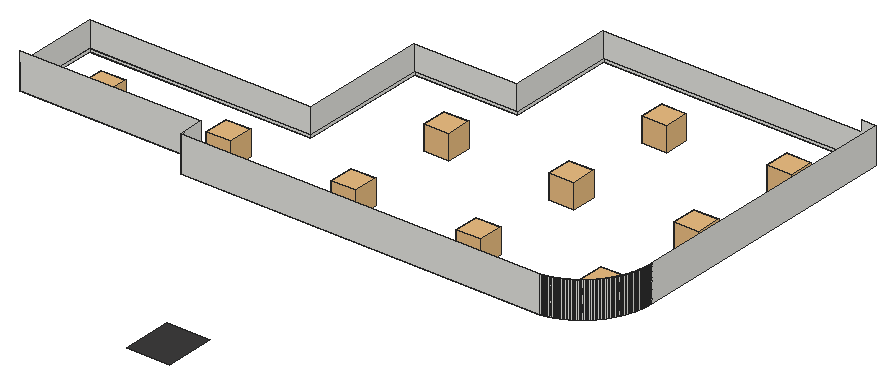
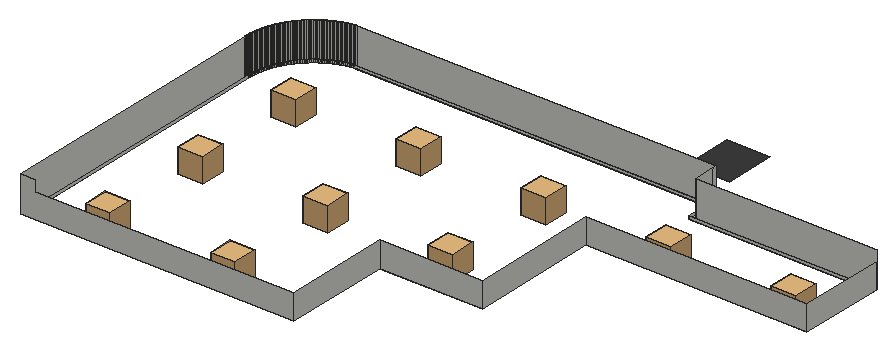
# SketchUp Ruby script. Lengths in inches.
U = 1.inch
M = Sketchup.active_model
def pt(a) = Geom::Point3d.new(a.map { |v| v * U })
def face(e, loops, mat)
  f = e.add_face(loops[0].map { |a| pt(a) })
  loops[1..].each { |l| e.add_face(l.map { |a| pt(a) }).erase! }
  f.material = f.back_material = mat if mat
  f
end
# faces: each face lists its corners as indices into pts; further lists are holes
def faces(e, pts, list, mat = nil) = list.each { |f| face(e, (f[0].is_a?(Array) ? f : [f]).map { |l| l.map { |i| pts[i] } }, mat) }
# xy, xz, yz: faces in a plane at the given z, y or x. An outline is a flat list of corners, or four numbers for a rectangle; further outlines are holes
def ring(l) = l.size == 4 ? [[l[0], l[1]], [l[2], l[1]], [l[2], l[3]], [l[0], l[3]]] : l.each_slice(2).to_a
def flat(e, list, mat, &to3) = list.each { |f| face(e, (f[0].is_a?(Array) ? f : [f]).map { |l| ring(l).map { |u, v| to3.(u, v) } }, mat) }
def xy(e, z, list, mat = nil) = flat(e, list, mat) { |x, y| [x, y, z] }
def xz(e, y, list, mat = nil) = flat(e, list, mat) { |x, z| [x, y, z] }
def yz(e, x, list, mat = nil) = flat(e, list, mat) { |y, z| [x, y, z] }
def lines(e, pts, list) = list.each { |a, b| e.add_line(pt(pts[a]), pt(pts[b])) }
# prism: a flat outline (further loops are holes) pulled along v
def prism(e, loops, v, mat = nil)
  f = face(e, loops, mat); d = Geom::Vector3d.new(v.map { |x| x * U })
  f.pushpull(f.normal.samedirection?(d) ? d.length : -d.length)
end
def box(e, o, s, mat = nil) = prism(e, [[o, [o[0] + s[0], o[1], o[2]], [o[0] + s[0], o[1] + s[1], o[2]], [o[0], o[1] + s[1], o[2]]]], [0, 0, s[2]], mat)
def at(x, y, z, deg = 0) = Geom::Transformation.translation(pt([x, y, z])) * Geom::Transformation.rotation(ORIGIN, Z_AXIS, deg.degrees)
def axes(o, x, y, z) = Geom::Transformation.new([*x, 0, *y, 0, *z, 0, *pt(o).to_a, 1])
def part(name) = M.definitions.add(name)
# library, detail: a bought-in or finely detailed component or shape, given as its bounding box
def library(name, o, s) = part(name).tap { |d| box(d.entities, o, s) }
def detail(e, o, s) = box(e.add_group.entities, o, s)
def put(e, d, t, mat = nil) = e.add_instance(d, t).tap { |i| i.material = mat if mat }
def group(e, t, mat = nil) = e.add_group.tap { |g| g.transformation = t; g.material = mat if mat }.entities
root = M.entities
M.materials.add("[Granite Dark Gray]").color = [61, 60, 60]
c1 = library("3",[-4.91,-4.91,-13.58],[13.82,13.82,13.58])
xy(root,75,[[168,58,192,86]],"[Granite Dark Gray]")
xy(root,106,[[[124.5,150,124.5,164,24,164,24,212,147,212,147,284,204,284,204,344,356,344,356,187.02,355.99,186.68,355.99,186.34,355.97,186.01,355.96,185.67,355.94,185.34,355.9,184.66,355.87,184.33,355.84,183.99,355.81,183.66,355.77,183.32,355.74,182.99,355.69,182.65,355.65,182.32,355.55,181.66,355.5,181.32,355.26,180,355.1875,179.67,355.12,179.34,355.04,179.01,354.97,178.68,354.89,178.36,354.81,178.03,354.72,177.7,354.54,177.06,354.45,176.73,354.15,175.77,353.93,175.13,353.82,174.8125,353.71,174.49,353.59,174.18,353.47,173.86,353.23,173.24,352.84,172.31,352.56,171.69,352.42,171.39,352.28,171.08,351.83,170.18,351.35,169.28,351.03,168.7,350.86,168.4,350.6875,168.11,350.52,167.83,350.16,167.25,349.98,166.97,349.8,166.6875,349.61,166.4,349.23,165.85,349.04,165.57,348.85,165.3,348.45,164.76,348.24,164.49,348.04,164.22,347.83,163.95,347.2,163.17,346.98,162.91,346.76,162.66,346.54,162.4,346.32,162.15,345.86,161.65,345.63,161.41,345.4,161.16,345.17,160.92,344.93,160.68,344.69,160.45,344.45,160.21,344.21,159.98,343.96,159.75,343.72,159.52,343.47,159.29,343.22,159.07,342.96,158.84,342.71,158.625,342.45,158.41,342.19,158.19,341.41,157.56,341.14,157.35,340.06,156.55,339.5,156.17,339.23,155.98,338.95,155.79,338.66,155.6,338.1,155.24,337.81,155.07,337.52,154.89,336.94,154.55,336.65,154.39,336.35,154.22,336.06,154.0625,335.76,153.9,335.46,153.75,335.16,153.59,334.86,153.44,334.5625,153.29,334.26,153.15,333.95,153.01,333.65,152.87,333.03,152.59,332.41,152.33,332.1,152.21,331.78,152.08,331.47,151.96,331.15,151.85,330.84,151.73,329.88,151.4,329.5625,151.3,329.24,151.2,328.6,151,328.27,150.91,327.95,150.82,327.625,150.73,327.3,150.65,326.64,150.49,326.31,150.42,325.99,150.34,325.66,150.28,325.33,150.21,325,150.15,324.66,150.09,324.17,150],[126.5,152,324,152,324.3125,152.05,324.63,152.11,325.25,152.23,325.57,152.3,325.88,152.37,326.1875,152.44,326.5,152.51,327.43,152.75,327.73,152.84,328.04,152.92,328.35,153.01,328.65,153.11,328.95,153.2,329.26,153.3,329.56,153.4,329.86,153.51,330.16,153.61,330.76,153.83,331.06,153.95,331.36,154.06,331.65,154.18,331.95,154.31,332.24,154.43,332.53,154.56,332.82,154.6875,333.11,154.82,333.4,154.96,333.6875,155.09,333.98,155.23,334.26,155.38,334.54,155.52,334.83,155.67,335.39,155.97,335.67,156.13,335.94,156.29,336.22,156.45,336.49,156.61,336.77,156.77,337.58,157.28,337.84,157.46,338.11,157.63,338.375,157.8125,338.64,158,338.9,158.18,339.15,158.37,339.41,158.55,339.67,158.75,339.92,158.9375,340.17,159.13,340.92,159.73,341.16,159.9375,341.41,160.14,341.65,160.35,341.89,160.5625,342.125,160.77,342.36,160.99,342.6,161.21,343.29,161.87,343.74,162.32,344.4,163.01,344.61,163.25,344.83,163.49,345.04,163.72,345.25,163.96,345.45,164.21,345.66,164.45,345.86,164.7,346.0625,164.94,346.26,165.19,346.46,165.44,346.65,165.7,346.84,165.95,347.41,166.73,347.77,167.25,347.95,167.52,348.125,167.78,348.3,168.05,348.64,168.59,348.8,168.86,348.97,169.13,349.13,169.41,349.29,169.6875,349.45,169.96,349.75,170.52,349.9,170.81,350.05,171.09,350.19,171.37,350.47,171.95,350.61,172.23,350.74,172.52,350.875,172.8125,351,173.11,351.13,173.4,351.25,173.69,351.37,173.99,351.49,174.28,351.61,174.58,351.83,175.18,351.9375,175.48,352.04,175.78,352.15,176.08,352.25,176.38,352.34,176.6875,352.4375,176.99,352.53,177.3,352.62,177.6,352.7,177.91,352.79,178.22,352.95,178.84,353.3,180.39,353.36,180.71,353.42,181.02,353.47,181.33,353.53,181.65,353.58,181.96,353.625,182.28,353.67,182.59,353.75,183.23,353.79,183.54,353.88,184.5,353.9,184.8125,353.93,185.13,353.95,185.45,353.96,185.77,353.98,186.09,353.99,186.41,354,186.72,354,342,206,342,206,282,149,282,149,210,26,210,26,166,126.5,166]]])
xz(root,150,[[124.5,106,324.17,126]])
xz(root,152,[[126.5,106,324,107.5]])
xz(root,164,[[24,106,124.5,126]])
xz(root,166,[[26,106,126.5,107.5]])
xz(root,210,[[26,106,149,107.5]])
xz(root,212,[[24,106,147,120]])
xz(root,282,[[149,106,206,107.5]])
xz(root,284,[[147,106,204,120]])
xz(root,342,[[206,106,354,107.5]])
xz(root,344,[[204,106,204,120,348,120,348,126,356,126,356,106]])
yz(root,24,[[164,106,212,120]])
yz(root,26,[[166,106,210,107.5]])
yz(root,124.5,[[150,106,152,126],[152,106,164,126]])
yz(root,126.5,[[152,106,166,107.5]])
yz(root,147,[[212,106,284,120]])
yz(root,149,[[210,106,282,107.5]])
yz(root,204,[[284,106,344,120]])
yz(root,206,[[282,106,342,107.5]])
yz(root,354,[[186.72,106,187.04,107.5],[187.04,106,187.36,107.5],[187.36,106,187.68,107.5],[187.68,106,188,107.5],[188,106,342,107.5]])
yz(root,355.99,[[186.34,106,186.68,126]])
yz(root,356,[[187.02,106,187.35,126],[187.35,106,187.69,126],[187.69,106,188.01,126],[188.01,106,344,126]])
p = [[324.66,150.09,126],[324.17,150,126],[324.17,150,106],[324.66,150.09,106],[325,150.15,126],[325,150.15,106],
  [325.33,150.21,126],[325.33,150.21,106],[325.66,150.28,126],[325.66,150.28,106],[325.99,150.34,126],[325.99,150.34,106],
  [326.31,150.42,126],[326.31,150.42,106],[326.64,150.49,126],[326.64,150.49,106],[326.97,150.57,126],[326.97,150.57,106],
  [327.3,150.65,126],[327.3,150.65,106],[327.625,150.73,126],[327.625,150.73,106],[327.95,150.82,126],[327.95,150.82,106],
  [328.27,150.91,126],[328.27,150.91,106],[328.6,151,126],[328.6,151,106],[328.92,151.1,126],[328.92,151.1,106],
  [329.24,151.2,126],[329.24,151.2,106],[329.5625,151.3,126],[329.5625,151.3,106],[329.88,151.4,126],[329.88,151.4,106],
  [330.2,151.51,126],[330.2,151.51,106],[330.52,151.62,126],[330.52,151.62,106],[330.84,151.73,126],[330.84,151.73,106],
  [331.15,151.85,126],[331.15,151.85,106],[331.47,151.96,126],[331.47,151.96,106],[324,152,107.5],[324.3125,152.05,107.5],
  [324.3125,152.05,106],[324,152,106],[331.78,152.08,126],[331.78,152.08,106],[324.63,152.11,107.5],[324.63,152.11,106],
  [324.94,152.17,107.5],[324.94,152.17,106],[332.1,152.21,126],[332.1,152.21,106],[325.25,152.23,107.5],[325.25,152.23,106],
  [325.57,152.3,107.5],[325.57,152.3,106],[332.41,152.33,126],[332.41,152.33,106],[325.88,152.37,107.5],[325.88,152.37,106],
  [332.72,152.46,126],[332.72,152.46,106],[326.1875,152.44,107.5],[326.1875,152.44,106],[326.5,152.51,107.5],[326.5,152.51,106],
  [326.81,152.59,107.5],[326.81,152.59,106],[333.03,152.59,126],[333.03,152.59,106],[327.12,152.67,107.5],[327.12,152.67,106],
  [333.34,152.73,126],[333.34,152.73,106],[327.43,152.75,107.5],[327.43,152.75,106],[333.65,152.87,126],[333.65,152.87,106],
  [327.73,152.84,107.5],[327.73,152.84,106],[328.04,152.92,107.5],[328.04,152.92,106],[328.35,153.01,107.5],[328.35,153.01,106],
  [333.95,153.01,126],[333.95,153.01,106],[328.65,153.11,107.5],[328.65,153.11,106],[334.26,153.15,126],[334.26,153.15,106],
  [328.95,153.2,107.5],[328.95,153.2,106],[334.5625,153.29,126],[334.5625,153.29,106],[329.26,153.3,107.5],[329.26,153.3,106],
  [329.56,153.4,107.5],[329.56,153.4,106],[334.86,153.44,126],[334.86,153.44,106],[329.86,153.51,107.5],[329.86,153.51,106],
  [335.16,153.59,126],[335.16,153.59,106],[330.16,153.61,107.5],[330.16,153.61,106],[330.46,153.72,107.5],[330.46,153.72,106],
  [335.46,153.75,126],[335.46,153.75,106],[330.76,153.83,107.5],[330.76,153.83,106],[335.76,153.9,126],[335.76,153.9,106],
  [331.06,153.95,107.5],[331.06,153.95,106],[331.36,154.06,107.5],[331.36,154.06,106],[336.06,154.0625,126],[336.06,154.0625,106],
  [331.65,154.18,107.5],[331.65,154.18,106],[336.35,154.22,126],[336.35,154.22,106],[331.95,154.31,107.5],[331.95,154.31,106],
  [336.65,154.39,126],[336.65,154.39,106],[332.24,154.43,107.5],[332.24,154.43,106],[332.53,154.56,107.5],[332.53,154.56,106],
  [336.94,154.55,126],[336.94,154.55,106],[332.82,154.6875,107.5],[332.82,154.6875,106],[337.23,154.72,126],[337.23,154.72,106],
  [333.11,154.82,107.5],[333.11,154.82,106],[337.52,154.89,126],[337.52,154.89,106],[333.4,154.96,107.5],[333.4,154.96,106],
  [337.81,155.07,126],[337.81,155.07,106],[333.6875,155.09,107.5],[333.6875,155.09,106],[333.98,155.23,107.5],[333.98,155.23,106],
  [338.1,155.24,126],[338.1,155.24,106],[334.26,155.38,107.5],[334.26,155.38,106],[338.38,155.42,126],[338.38,155.42,106],
  [334.54,155.52,107.5],[334.54,155.52,106],[338.66,155.6,126],[338.66,155.6,106],[334.83,155.67,107.5],[334.83,155.67,106],
  [338.95,155.79,126],[338.95,155.79,106],[335.11,155.82,107.5],[335.11,155.82,106],[335.39,155.97,107.5],[335.39,155.97,106],
  [339.23,155.98,126],[339.23,155.98,106],[335.67,156.13,107.5],[335.67,156.13,106],[339.5,156.17,126],[339.5,156.17,106],
  [335.94,156.29,107.5],[335.94,156.29,106],[339.78,156.36,126],[339.78,156.36,106],[336.22,156.45,107.5],[336.22,156.45,106],
  [336.49,156.61,107.5],[336.49,156.61,106],[340.06,156.55,126],[340.06,156.55,106],[336.77,156.77,107.5],[336.77,156.77,106],
  [340.33,156.75,126],[340.33,156.75,106],[340.6,156.95,126],[340.6,156.95,106],[337.04,156.94,107.5],[337.04,156.94,106],
  [337.31,157.11,107.5],[337.31,157.11,106],[340.87,157.15,126],[340.87,157.15,106],[337.58,157.28,107.5],[337.58,157.28,106],
  [341.14,157.35,126],[341.14,157.35,106],[337.84,157.46,107.5],[337.84,157.46,106],[341.41,157.56,126],[341.41,157.56,106],
  [338.11,157.63,107.5],[338.11,157.63,106],[338.375,157.8125,107.5],[338.375,157.8125,106],[341.67,157.77,126],[341.67,157.77,106],
  [338.64,158,107.5],[338.64,158,106],[341.93,157.98,126],[341.93,157.98,106],[338.9,158.18,107.5],[338.9,158.18,106],
  [342.19,158.19,126],[342.19,158.19,106],[339.15,158.37,107.5],[339.15,158.37,106],[342.45,158.41,126],[342.45,158.41,106],
  [339.41,158.55,107.5],[339.41,158.55,106],[342.71,158.625,126],[342.71,158.625,106],[339.67,158.75,107.5],[339.67,158.75,106],
  [342.96,158.84,126],[342.96,158.84,106],[339.92,158.9375,107.5],[339.92,158.9375,106],[343.22,159.07,126],[343.22,159.07,106],
  [340.17,159.13,107.5],[340.17,159.13,106],[340.42,159.33,107.5],[340.42,159.33,106],[343.47,159.29,126],[343.47,159.29,106],
  [340.67,159.53,107.5],[340.67,159.53,106],[343.72,159.52,126],[343.72,159.52,106],[340.92,159.73,107.5],[340.92,159.73,106],
  [343.96,159.75,126],[343.96,159.75,106],[341.16,159.9375,107.5],[341.16,159.9375,106],[344.21,159.98,126],[344.21,159.98,106],
  [341.41,160.14,107.5],[341.41,160.14,106],[344.45,160.21,126],[344.45,160.21,106],[341.65,160.35,107.5],[341.65,160.35,106],
  [344.69,160.45,126],[344.69,160.45,106],[341.89,160.5625,107.5],[341.89,160.5625,106],[344.93,160.68,126],[344.93,160.68,106],
  [342.125,160.77,107.5],[342.125,160.77,106],[345.17,160.92,126],[345.17,160.92,106],[342.36,160.99,107.5],[342.36,160.99,106],
  [345.4,161.16,126],[345.4,161.16,106],[342.6,161.21,107.5],[342.6,161.21,106],[342.83,161.43,107.5],[342.83,161.43,106],
  [345.63,161.41,126],[345.63,161.41,106],[343.06,161.65,107.5],[343.06,161.65,106],[345.86,161.65,126],[345.86,161.65,106],
  [343.29,161.87,107.5],[343.29,161.87,106],[346.09,161.9,126],[346.09,161.9,106],[343.51,162.09,107.5],[343.51,162.09,106],
  [346.32,162.15,126],[346.32,162.15,106],[343.74,162.32,107.5],[343.74,162.32,106],[346.54,162.4,126],[346.54,162.4,106],
  [343.96,162.55,107.5],[343.96,162.55,106],[346.76,162.66,126],[346.76,162.66,106],[344.18,162.78,107.5],[344.18,162.78,106],
  [346.98,162.91,126],[346.98,162.91,106],[344.4,163.01,107.5],[344.4,163.01,106],[347.2,163.17,126],[347.2,163.17,106],
  [344.61,163.25,107.5],[344.61,163.25,106],[344.83,163.49,107.5],[344.83,163.49,106],[347.41,163.43,126],[347.41,163.43,106],
  [347.62,163.69,126],[347.62,163.69,106],[345.04,163.72,107.5],[345.04,163.72,106],[345.25,163.96,107.5],[345.25,163.96,106],
  [347.83,163.95,126],[347.83,163.95,106],[345.45,164.21,107.5],[345.45,164.21,106],[348.04,164.22,126],[348.04,164.22,106],
  [345.66,164.45,107.5],[345.66,164.45,106],[348.24,164.49,126],[348.24,164.49,106],[345.86,164.7,107.5],[345.86,164.7,106],
  [348.45,164.76,126],[348.45,164.76,106],[346.0625,164.94,107.5],[346.0625,164.94,106],[348.65,165.03,126],[348.65,165.03,106],
  [346.26,165.19,107.5],[346.26,165.19,106],[348.85,165.3,126],[348.85,165.3,106],[346.46,165.44,107.5],[346.46,165.44,106],
  [349.04,165.57,126],[349.04,165.57,106],[346.65,165.7,107.5],[346.65,165.7,106],[349.23,165.85,126],[349.23,165.85,106],
  [346.84,165.95,107.5],[346.84,165.95,106],[349.42,166.125,126],[349.42,166.125,106],[347.03,166.21,107.5],[347.03,166.21,106],
  [349.61,166.4,126],[349.61,166.4,106],[347.22,166.47,107.5],[347.22,166.47,106],[349.8,166.6875,126],[349.8,166.6875,106],
  [347.41,166.73,107.5],[347.41,166.73,106],[347.59,166.99,107.5],[347.59,166.99,106],[349.98,166.97,126],[349.98,166.97,106],
  [347.77,167.25,107.5],[347.77,167.25,106],[350.16,167.25,126],[350.16,167.25,106],[347.95,167.52,107.5],[347.95,167.52,106],
  [350.34,167.54,126],[350.34,167.54,106],[348.125,167.78,107.5],[348.125,167.78,106],[350.52,167.83,126],[350.52,167.83,106],
  [348.3,168.05,107.5],[348.3,168.05,106],[350.6875,168.11,126],[350.6875,168.11,106],[348.47,168.32,107.5],[348.47,168.32,106],
  [350.86,168.4,126],[350.86,168.4,106],[348.64,168.59,107.5],[348.64,168.59,106],[351.03,168.7,126],[351.03,168.7,106],
  [348.8,168.86,107.5],[348.8,168.86,106],[351.19,168.99,126],[351.19,168.99,106],[348.97,169.13,107.5],[348.97,169.13,106],
  [351.35,169.28,126],[351.35,169.28,106],[349.13,169.41,107.5],[349.13,169.41,106],[351.51,169.58,126],[351.51,169.58,106],
  [349.29,169.6875,107.5],[349.29,169.6875,106],[351.67,169.88,126],[351.67,169.88,106],[349.45,169.96,107.5],[349.45,169.96,106],
  [351.83,170.18,126],[351.83,170.18,106],[349.6,170.24,107.5],[349.6,170.24,106],[349.75,170.52,107.5],[349.75,170.52,106],
  [351.98,170.48,126],[351.98,170.48,106],[349.9,170.81,107.5],[349.9,170.81,106],[352.13,170.78,126],[352.13,170.78,106],
  [350.05,171.09,107.5],[350.05,171.09,106],[352.28,171.08,126],[352.28,171.08,106],[350.19,171.37,107.5],[350.19,171.37,106],
  [352.42,171.39,126],[352.42,171.39,106],[350.33,171.66,107.5],[350.33,171.66,106],[352.56,171.69,126],[352.56,171.69,106],
  [350.47,171.95,107.5],[350.47,171.95,106],[352.7,172,126],[352.7,172,106],[350.61,172.23,107.5],[350.61,172.23,106],
  [352.84,172.31,126],[352.84,172.31,106],[350.74,172.52,107.5],[350.74,172.52,106],[352.97,172.62,126],[352.97,172.62,106],
  [350.875,172.8125,107.5],[350.875,172.8125,106],[353.1,172.93,126],[353.1,172.93,106],[351,173.11,107.5],[351,173.11,106],
  [353.23,173.24,126],[353.23,173.24,106],[351.13,173.4,107.5],[351.13,173.4,106],[353.35,173.55,126],[353.35,173.55,106],
  [351.25,173.69,107.5],[351.25,173.69,106],[353.47,173.86,126],[353.47,173.86,106],[351.37,173.99,107.5],[351.37,173.99,106],
  [353.59,174.18,126],[353.59,174.18,106],[351.49,174.28,107.5],[351.49,174.28,106],[353.71,174.49,126],[353.71,174.49,106],
  [351.61,174.58,107.5],[351.61,174.58,106],[353.82,174.8125,126],[353.82,174.8125,106],[351.72,174.88,107.5],[351.72,174.88,106],
  [353.93,175.13,126],[353.93,175.13,106],[351.83,175.18,107.5],[351.83,175.18,106],[354.04,175.45,126],[354.04,175.45,106],
  [351.9375,175.48,107.5],[351.9375,175.48,106],[354.15,175.77,126],[354.15,175.77,106],[352.04,175.78,107.5],[352.04,175.78,106],
  [352.15,176.08,107.5],[352.15,176.08,106],[354.25,176.09,126],[354.25,176.09,106],[352.25,176.38,107.5],[352.25,176.38,106],
  [354.35,176.41,126],[354.35,176.41,106],[352.34,176.6875,107.5],[352.34,176.6875,106],[354.45,176.73,126],[354.45,176.73,106],
  [352.4375,176.99,107.5],[352.4375,176.99,106],[354.54,177.06,126],[354.54,177.06,106],[352.53,177.3,107.5],[352.53,177.3,106],
  [354.63,177.38,126],[354.63,177.38,106],[352.62,177.6,107.5],[352.62,177.6,106],[354.72,177.7,126],[354.72,177.7,106],
  [352.7,177.91,107.5],[352.7,177.91,106],[354.81,178.03,126],[354.81,178.03,106],[352.79,178.22,107.5],[352.79,178.22,106],
  [354.89,178.36,126],[354.89,178.36,106],[352.87,178.53,107.5],[352.87,178.53,106],[354.97,178.68,126],[354.97,178.68,106],
  [352.95,178.84,107.5],[352.95,178.84,106],[355.04,179.01,126],[355.04,179.01,106],[353.02,179.15,107.5],[353.02,179.15,106],
  [355.12,179.34,126],[355.12,179.34,106],[353.09,179.46,107.5],[353.09,179.46,106],[355.1875,179.67,126],[355.1875,179.67,106],
  [353.16,179.77,107.5],[353.16,179.77,106],[355.26,180,126],[355.26,180,106],[353.23,180.08,107.5],[353.23,180.08,106],
  [355.32,180.33,126],[355.32,180.33,106],[353.3,180.39,107.5],[353.3,180.39,106],[355.38,180.66,126],[355.38,180.66,106],
  [353.36,180.71,107.5],[353.36,180.71,106],[353.42,181.02,107.5],[353.42,181.02,106],[355.44,180.99,126],[355.44,180.99,106],
  [353.47,181.33,107.5],[353.47,181.33,106],[355.5,181.32,126],[355.5,181.32,106],[353.53,181.65,107.5],[353.53,181.65,106],
  [355.55,181.66,126],[355.55,181.66,106],[353.58,181.96,107.5],[353.58,181.96,106],[355.6,181.99,126],[355.6,181.99,106],
  [353.625,182.28,107.5],[353.625,182.28,106],[355.65,182.32,126],[355.65,182.32,106],[353.67,182.59,107.5],[353.67,182.59,106],
  [355.69,182.65,126],[355.69,182.65,106],[353.71,182.91,107.5],[353.71,182.91,106],[355.74,182.99,126],[355.74,182.99,106],
  [353.75,183.23,107.5],[353.75,183.23,106],[355.77,183.32,126],[355.77,183.32,106],[353.79,183.54,107.5],[353.79,183.54,106],
  [355.81,183.66,126],[355.81,183.66,106],[353.82,183.86,107.5],[353.82,183.86,106],[355.84,183.99,126],[355.84,183.99,106],
  [353.85,184.18,107.5],[353.85,184.18,106],[355.87,184.33,126],[355.87,184.33,106],[353.88,184.5,107.5],[353.88,184.5,106],
  [355.9,184.66,126],[355.9,184.66,106],[353.9,184.8125,107.5],[353.9,184.8125,106],[355.92,185,126],[355.92,185,106],
  [353.93,185.13,107.5],[353.93,185.13,106],[355.94,185.34,126],[355.94,185.34,106],[353.95,185.45,107.5],[353.95,185.45,106],
  [355.96,185.67,126],[355.96,185.67,106],[353.96,185.77,107.5],[353.96,185.77,106],[355.97,186.01,126],[355.97,186.01,106],
  [353.98,186.09,107.5],[353.98,186.09,106],[355.99,186.34,126],[355.99,186.34,106],[353.99,186.41,107.5],[353.99,186.41,106],
  [354,186.72,107.5],[354,186.72,106],[356,187.02,126],[355.99,186.68,126],[355.99,186.68,106],[356,187.02,106]]
faces(root,p,[[0,1,2,3],[4,0,3,5],[6,4,5,7],[8,6,7,9],[10,8,9,11],[12,10,11,13],[14,12,13,15],[16,14,15,17],
  [18,16,17,19],[20,18,19,21],[22,20,21,23],[24,22,23,25],[26,24,25,27],[28,26,27,29],[30,28,29,31],[32,30,31,33],
  [34,32,33,35],[36,34,35,37],[38,36,37,39],[40,38,39,41],[42,40,41,43],[44,42,43,45],[46,47,48,49],[50,44,45,51],
  [47,52,53,48],[52,54,55,53],[56,50,51,57],[54,58,59,55],[58,60,61,59],[62,56,57,63],[60,64,65,61],[66,62,63,67],
  [64,68,69,65],[68,70,71,69],[70,72,73,71],[74,66,67,75],[72,76,77,73],[78,74,75,79],[76,80,81,77],[82,78,79,83],
  [80,84,85,81],[84,86,87,85],[86,88,89,87],[90,82,83,91],[88,92,93,89],[94,90,91,95],[92,96,97,93],[98,94,95,99],
  [96,100,101,97],[100,102,103,101],[104,98,99,105],[102,106,107,103],[108,104,105,109],[106,110,111,107],[110,112,113,111],[114,108,109,115],
  [112,116,117,113],[118,114,115,119],[116,120,121,117],[120,122,123,121],[124,118,119,125],[122,126,127,123],[128,124,125,129],[126,130,131,127],
  [132,128,129,133],[130,134,135,131],[134,136,137,135],[138,132,133,139],[136,140,141,137],[142,138,139,143],[140,144,145,141],[146,142,143,147],
  [144,148,149,145],[150,146,147,151],[148,152,153,149],[152,154,155,153],[156,150,151,157],[154,158,159,155],[160,156,157,161],[158,162,163,159],
  [164,160,161,165],[162,166,167,163],[168,164,165,169],[166,170,171,167],[170,172,173,171],[174,168,169,175],[172,176,177,173],[178,174,175,179],
  [176,180,181,177],[182,178,179,183],[180,184,185,181],[184,186,187,185],[188,182,183,189],[186,190,191,187],[192,188,189,193],[194,192,193,195],
  [190,196,197,191],[196,198,199,197],[200,194,195,201],[198,202,203,199],[204,200,201,205],[202,206,207,203],[208,204,205,209],[206,210,211,207],
  [210,212,213,211],[214,208,209,215],[212,216,217,213],[218,214,215,219],[216,220,221,217],[222,218,219,223],[220,224,225,221],[226,222,223,227],
  [224,228,229,225],[230,226,227,231],[228,232,233,229],[234,230,231,235],[232,236,237,233],[238,234,235,239],[236,240,241,237],[240,242,243,241],
  [244,238,239,245],[242,246,247,243],[248,244,245,249],[246,250,251,247],[252,248,249,253],[250,254,255,251],[256,252,253,257],[254,258,259,255],
  [260,256,257,261],[258,262,263,259],[264,260,261,265],[262,266,267,263],[268,264,265,269],[266,270,271,267],[272,268,269,273],[270,274,275,271],
  [276,272,273,277],[274,278,279,275],[278,280,281,279],[282,276,277,283],[280,284,285,281],[286,282,283,287],[284,288,289,285],[290,286,287,291],
  [288,292,293,289],[294,290,291,295],[292,296,297,293],[298,294,295,299],[296,300,301,297],[302,298,299,303],[300,304,305,301],[306,302,303,307],
  [304,308,309,305],[310,306,307,311],[308,312,313,309],[312,314,315,313],[316,310,311,317],[318,316,317,319],[314,320,321,315],[320,322,323,321],
  [324,318,319,325],[322,326,327,323],[328,324,325,329],[326,330,331,327],[332,328,329,333],[330,334,335,331],[336,332,333,337],[334,338,339,335],
  [340,336,337,341],[338,342,343,339],[344,340,341,345],[342,346,347,343],[348,344,345,349],[346,350,351,347],[352,348,349,353],[350,354,355,351],
  [356,352,353,357],[354,358,359,355],[360,356,357,361],[358,362,363,359],[364,360,361,365],[362,366,367,363],[366,368,369,367],[370,364,365,371],
  [368,372,373,369],[374,370,371,375],[372,376,377,373],[378,374,375,379],[376,380,381,377],[382,378,379,383],[380,384,385,381],[386,382,383,387],
  [384,388,389,385],[390,386,387,391],[388,392,393,389],[394,390,391,395],[392,396,397,393],[398,394,395,399],[396,400,401,397],[402,398,399,403],
  [400,404,405,401],[406,402,403,407],[404,408,409,405],[410,406,407,411],[408,412,413,409],[414,410,411,415],[412,416,417,413],[416,418,419,417],
  [420,414,415,421],[418,422,423,419],[424,420,421,425],[422,426,427,423],[428,424,425,429],[426,430,431,427],[432,428,429,433],[430,434,435,431],
  [436,432,433,437],[434,438,439,435],[440,436,437,441],[438,442,443,439],[444,440,441,445],[442,446,447,443],[448,444,445,449],[446,450,451,447],
  [452,448,449,453],[450,454,455,451],[456,452,453,457],[454,458,459,455],[460,456,457,461],[458,462,463,459],[464,460,461,465],[462,466,467,463],
  [468,464,465,469],[466,470,471,467],[472,468,469,473],[470,474,475,471],[476,472,473,477],[474,478,479,475],[480,476,477,481],[478,482,483,479],
  [484,480,481,485],[482,486,487,483],[488,484,485,489],[486,490,491,487],[490,492,493,491],[494,488,489,495],[492,496,497,493],[498,494,495,499],
  [496,500,501,497],[502,498,499,503],[500,504,505,501],[506,502,503,507],[504,508,509,505],[510,506,507,511],[508,512,513,509],[514,510,511,515],
  [512,516,517,513],[518,514,515,519],[516,520,521,517],[522,518,519,523],[520,524,525,521],[526,522,523,527],[524,528,529,525],[530,526,527,531],
  [528,532,533,529],[534,530,531,535],[532,536,537,533],[538,534,535,539],[536,540,541,537],[542,538,539,543],[540,544,545,541],[546,542,543,547],
  [544,548,549,545],[550,546,547,551],[548,552,553,549],[552,554,555,553],[556,550,551,557],[554,558,559,555],[560,556,557,561],[558,562,563,559],
  [564,560,561,565],[562,566,567,563],[568,564,565,569],[566,570,571,567],[572,568,569,573],[570,574,575,571],[576,572,573,577],[574,578,579,575],
  [580,576,577,581],[578,582,583,579],[584,580,581,585],[582,586,587,583],[588,584,585,589],[586,590,591,587],[592,588,589,593],[590,594,595,591],
  [596,592,593,597],[594,598,599,595],[600,596,597,601],[598,602,603,599],[604,600,601,605],[602,606,607,603],[608,604,605,609],[606,610,611,607],
  [612,608,609,613],[610,614,615,611],[616,612,613,617],[614,618,619,615],[620,616,617,621],[618,622,623,619],[622,624,625,623],[626,627,628,629]])
put(root,c1,at(257.5,186,109.5))
put(root,c1,at(327,186,109.5))
put(root,c1,at(257.5,250.5,109.5))
put(root,c1,at(327,250.5,109.5))
put(root,c1,at(188,250.5,109.5))
put(root,c1,at(257.5,315,109.5))
put(root,c1,at(327,315,109.5))
put(root,c1,at(188,186,109.5))
put(root,c1,at(49,186,109.5))
put(root,c1,at(118.5,186,109.5))
